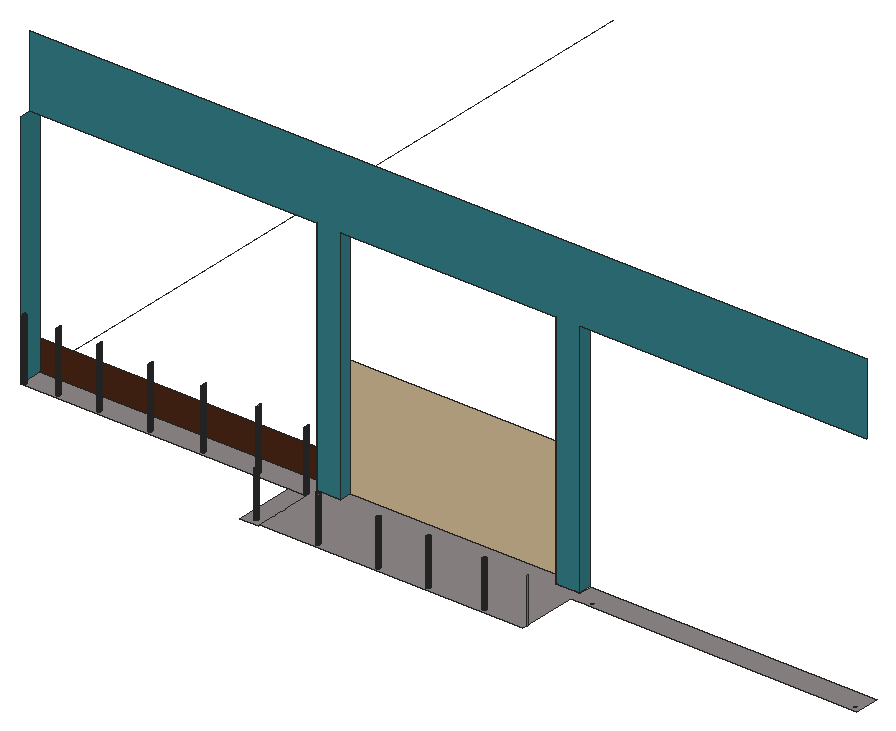
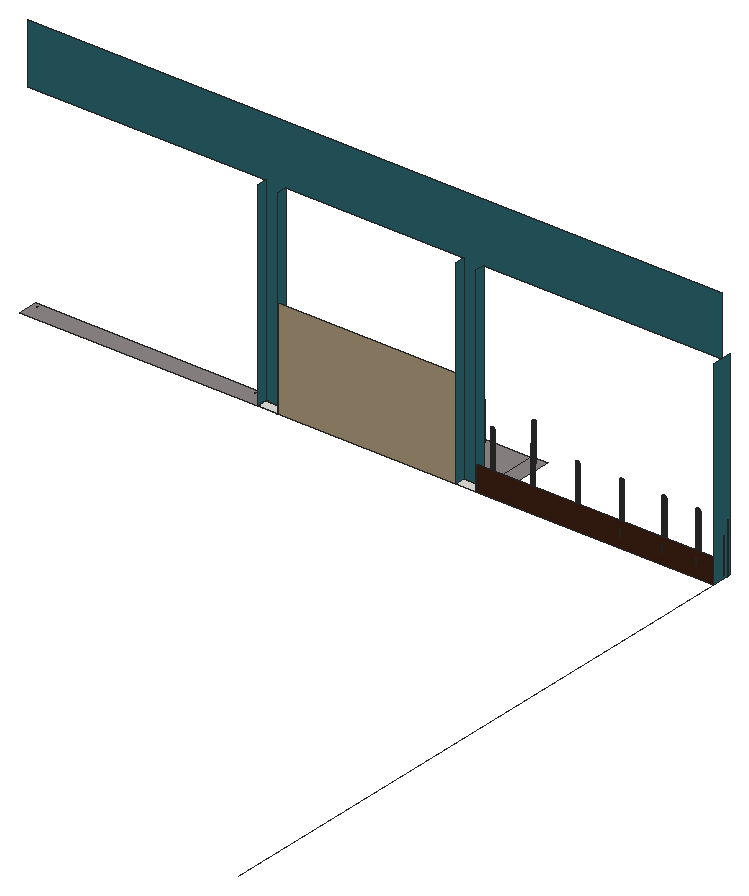
# SketchUp Ruby script. Lengths in inches.
U = 1.inch
M = Sketchup.active_model
def pt(a) = Geom::Point3d.new(a.map { |v| v * U })
def face(e, loops, mat)
  f = e.add_face(loops[0].map { |a| pt(a) })
  loops[1..].each { |l| e.add_face(l.map { |a| pt(a) }).erase! }
  f.material = f.back_material = mat if mat
  f
end
# faces: each face lists its corners as indices into pts; further lists are holes
def faces(e, pts, list, mat = nil) = list.each { |f| face(e, (f[0].is_a?(Array) ? f : [f]).map { |l| l.map { |i| pts[i] } }, mat) }
# xy, xz, yz: faces in a plane at the given z, y or x. An outline is a flat list of corners, or four numbers for a rectangle; further outlines are holes
def ring(l) = l.size == 4 ? [[l[0], l[1]], [l[2], l[1]], [l[2], l[3]], [l[0], l[3]]] : l.each_slice(2).to_a
def flat(e, list, mat, &to3) = list.each { |f| face(e, (f[0].is_a?(Array) ? f : [f]).map { |l| ring(l).map { |u, v| to3.(u, v) } }, mat) }
def xy(e, z, list, mat = nil) = flat(e, list, mat) { |x, y| [x, y, z] }
def xz(e, y, list, mat = nil) = flat(e, list, mat) { |x, z| [x, y, z] }
def yz(e, x, list, mat = nil) = flat(e, list, mat) { |y, z| [x, y, z] }
def lines(e, pts, list) = list.each { |a, b| e.add_line(pt(pts[a]), pt(pts[b])) }
# prism: a flat outline (further loops are holes) pulled along v
def prism(e, loops, v, mat = nil)
  f = face(e, loops, mat); d = Geom::Vector3d.new(v.map { |x| x * U })
  f.pushpull(f.normal.samedirection?(d) ? d.length : -d.length)
end
def box(e, o, s, mat = nil) = prism(e, [[o, [o[0] + s[0], o[1], o[2]], [o[0] + s[0], o[1] + s[1], o[2]], [o[0], o[1] + s[1], o[2]]]], [0, 0, s[2]], mat)
def at(x, y, z, deg = 0) = Geom::Transformation.translation(pt([x, y, z])) * Geom::Transformation.rotation(ORIGIN, Z_AXIS, deg.degrees)
def axes(o, x, y, z) = Geom::Transformation.new([*x, 0, *y, 0, *z, 0, *pt(o).to_a, 1])
def part(name) = M.definitions.add(name)
# library, detail: a bought-in or finely detailed component or shape, given as its bounding box
def library(name, o, s) = part(name).tap { |d| box(d.entities, o, s) }
def detail(e, o, s) = box(e.add_group.entities, o, s)
def put(e, d, t, mat = nil) = e.add_instance(d, t).tap { |i| i.material = mat if mat }
def group(e, t, mat = nil) = e.add_group.tap { |g| g.transformation = t; g.material = mat if mat }.entities
root = M.entities
M.materials.add("[0032_Moccasin]").color = [214, 191, 152]
M.materials.add("[0042_Sienna]").color = [76, 39, 21]
M.materials.add("[0083_DarkTurquoise]").color = [52, 127, 137]
M.materials.add("[Steel Brushed Stainless]").color = [183, 187, 190]
M.materials.add("[Stone Marble]").color = [143, 138, 136]
xy(root,167.95,[[648,109.2,672,121.2]])
xy(root,168,[[404.47,98.37,403.95,98.43,403.47,98.63,403.06,98.95,402.74,99.37,402.54,99.85,402.47,100.37,402.54,100.88,402.74,101.37,403.06,101.78,403.47,102.1,403.95,102.3,404.47,102.37,404.99,102.3,405.47,102.1,405.89,101.78,406.2,101.37,406.4,100.88,406.47,100.37,406.4,99.85,406.2,99.37,405.89,98.95,405.47,98.63,404.99,98.43],[408,109.2,432,121.2],[648,109.2,672,121.2]])
xy(root,168,[[[389.3,36.24,408,97.2],[400.07,41.47,399.55,41.54,399.07,41.74,398.65,42.05,398.33,42.47,398.13,42.95,398.07,43.47,398.13,43.99,398.33,44.47,398.65,44.88,399.07,45.2,399.55,45.4,400.07,45.47,400.58,45.4,401.07,45.2,401.48,44.88,401.8,44.47,402,43.99,402.07,43.47,402,42.95,401.8,42.47,401.48,42.05,401.07,41.74,400.58,41.54]],[[408,37.2,672,37.2,672,98.16,690.7,98.16,690.7,97.2,960,97.2,960,121.2,672,121.2,672,109.2,648,109.2,648,121.2,432,121.2,432,109.2,408,109.2,408,121.2,120,121.2,120,100.88,120.2,101.37,120.52,101.78,120.93,102.1,121.41,102.3,121.93,102.37,122.45,102.3,122.93,102.1,123.35,101.78,123.66,101.37,123.86,100.88,123.93,100.37,123.86,99.85,123.66,99.37,123.35,98.95,122.93,98.63,122.45,98.43,121.93,98.37,121.41,98.43,120.93,98.63,120.52,98.95,120.2,99.37,120,99.85,120,97.2,408,97.2],[954.01,100.13,953.77,100.17,953.53,100.2,953.51,100.21,953.49,100.21,953.05,100.39,953.03,100.41,953.01,100.41,952.82,100.5625,952.63,100.7,952.62,100.72,952.6,100.74,952.46,100.93,952.31,101.12,952.3,101.14,952.29,101.15,952.2,101.375,952.1,101.6,952.1,101.62,952.09,101.64,952.0625,101.875,952.03,102.11,952.03,102.16,952.0625,102.39,952.09,102.63,952.1,102.65,952.1,102.67,952.2,102.89,952.29,103.12,952.3,103.13,952.31,103.15,952.46,103.34,952.6,103.53,952.63,103.56,953.01,103.86,953.03,103.86,953.05,103.88,953.27,103.97,953.49,104.0625,953.51,104.0625,953.53,104.07,954.01,104.13,954.05,104.13,954.29,104.1,954.52,104.07,954.55,104.0625,954.57,104.0625,954.79,103.97,955.01,103.88,955.03,103.86,955.05,103.86,955.43,103.56,955.46,103.53,955.6,103.34,955.75,103.15,955.76,103.13,955.77,103.12,955.86,102.89,955.95,102.67,955.97,102.63,955.99,102.39,956.03,102.16,956.03,102.11,955.99,101.875,955.97,101.64,955.95,101.6,955.77,101.15,955.76,101.14,955.75,101.12,955.6,100.93,955.46,100.74,955.44,100.72,955.43,100.7,955.24,100.5625,955.05,100.41,955.03,100.41,955.01,100.39,954.57,100.21,954.55,100.21,954.52,100.2,954.29,100.17,954.05,100.13,954.03,100.14],[690.43,100.13,689.91,100.2,689.42,100.39,689.01,100.7,688.68,101.12,688.48,101.6,688.4,102.11,688.47,102.63,688.66,103.12,688.97,103.53,689.38,103.86,689.86,104.0625,690.38,104.13,690.9,104.07,691.38,103.88,691.8,103.56,692.125,103.15,692.33,102.67,692.4,102.16,692.34,101.64,692.15,101.15,691.83,100.74,691.42,100.41,690.94,100.21],[404.47,98.37,403.95,98.43,403.47,98.63,403.06,98.95,402.74,99.37,402.54,99.85,402.47,100.37,402.54,100.88,402.74,101.37,403.06,101.78,403.47,102.1,403.95,102.3,404.47,102.37,404.99,102.3,405.47,102.1,405.89,101.78,406.2,101.37,406.4,100.88,406.47,100.37,406.4,99.85,406.2,99.37,405.89,98.95,405.47,98.63,404.99,98.43]],[400.07,41.47,399.55,41.54,399.07,41.74,398.65,42.05,398.33,42.47,398.13,42.95,398.07,43.47,398.13,43.99,398.33,44.47,398.65,44.88,399.07,45.2,399.55,45.4,400.07,45.47,400.58,45.4,401.07,45.2,401.48,44.88,401.8,44.47,402,43.99,402.07,43.47,402,42.95,401.8,42.47,401.48,42.05,401.07,41.74,400.58,41.54]],"[Stone Marble]")
xz(root,109.2,[[648,167.95,672,168]])
xz(root,109.2,[[408,168,432,168,432,408,648,408,648,168,672,168,672,408,960,408,960,480,120,480,120,408,408,408]],"[0083_DarkTurquoise]")
xz(root,121.2,[[648,167.95,672,168]])
xz(root,121.2,[[432,168,648,288]],"[0032_Moccasin]")
xz(root,121.2,[[120,168,408,198]],"[0042_Sienna]")
yz(root,120,[[97.2,168,121.2,408]],"[0083_DarkTurquoise]")
yz(root,408,[[109.2,168,121.2,408]],"[0083_DarkTurquoise]")
yz(root,432,[[109.2,168,121.2,408]],"[0083_DarkTurquoise]")
yz(root,648,[[109.2,167.95,121.2,168]])
yz(root,648,[[109.2,168,121.2,408]],"[0083_DarkTurquoise]")
yz(root,672,[[109.2,167.95,121.2,168]])
yz(root,672,[[109.2,168,121.2,408]],"[0083_DarkTurquoise]")
p = [[461.31,41.04,168],[461.79,40.84,168],[461.79,40.84,213.56],[461.31,41.04,213.56],[462.31,40.78,168],[462.31,40.78,213.56],
  [462.83,40.84,168],[462.83,40.84,213.56],[463.31,41.04,168],[463.31,41.04,213.56],[522.25,41.04,168],[522.73,40.84,168],
  [522.73,40.84,213.56],[522.25,41.04,213.56],[523.25,40.78,168],[523.25,40.78,213.56],[523.76,40.84,168],[523.76,40.84,213.56],
  [524.25,41.04,168],[524.25,41.04,213.56],[572.31,41.04,168],[572.79,40.84,168],[572.79,40.84,213.56],[572.31,41.04,213.56],
  [573.31,40.78,168],[573.31,40.78,213.56],[573.83,40.84,168],[573.83,40.84,213.56],[574.31,41.04,168],[574.31,41.04,213.56],
  [628.68,41.04,168],[629.17,40.84,168],[629.17,40.84,213.56],[628.68,41.04,213.56],[629.68,40.78,168],[629.68,40.78,213.56],
  [630.2,40.84,168],[630.2,40.84,213.56],[630.68,41.04,168],[630.68,41.04,213.56],[460.89,41.36,168],[460.89,41.36,213.56],
  [463.72,41.36,168],[463.72,41.36,213.56],[521.83,41.36,168],[521.83,41.36,213.56],[524.66,41.36,168],[524.66,41.36,213.56],
  [571.89,41.36,168],[571.89,41.36,213.56],[574.72,41.36,168],[574.72,41.36,213.56],[628.27,41.36,168],[628.27,41.36,213.56],
  [631.1,41.36,168],[631.1,41.36,213.56],[460.58,41.78,168],[460.58,41.78,213.56],[464.04,41.78,168],[464.04,41.78,213.56],
  [521.51,41.78,168],[521.51,41.78,213.56],[524.98,41.78,168],[524.98,41.78,213.56],[571.58,41.78,168],[571.58,41.78,213.56],
  [575.04,41.78,168],[575.04,41.78,213.56],[627.95,41.78,168],[627.95,41.78,213.56],[631.41,41.78,168],[631.41,41.78,213.56],
  [399.07,41.74,168],[399.55,41.54,168],[399.55,41.54,213.19],[399.07,41.74,213.19],[400.07,41.47,168],[400.07,41.47,213.19],
  [400.58,41.54,168],[400.58,41.54,213.19],[401.07,41.74,168],[401.07,41.74,213.19],[398.65,42.05,168],[398.65,42.05,213.19],
  [401.48,42.05,168],[401.48,42.05,213.19],[460.375,42.26,168],[460.375,42.26,213.56],[464.24,42.26,168],[464.24,42.26,213.56],
  [521.3125,42.26,168],[521.3125,42.26,213.56],[525.18,42.26,168],[525.18,42.26,213.56],[571.375,42.26,168],[571.375,42.26,213.56],
  [575.24,42.26,168],[575.24,42.26,213.56],[627.75,42.26,168],[627.75,42.26,213.56],[631.61,42.26,168],[631.61,42.26,213.56],
  [398.33,42.47,168],[398.33,42.47,213.19],[401.8,42.47,168],[401.8,42.47,213.19],[460.31,42.78,168],[460.31,42.78,213.56],
  [464.31,42.78,168],[464.31,42.78,213.56],[521.25,42.78,168],[521.25,42.78,213.56],[525.25,42.78,168],[525.25,42.78,213.56],
  [571.31,42.78,168],[571.31,42.78,213.56],[575.31,42.78,168],[575.31,42.78,213.56],[627.68,42.78,168],[627.68,42.78,213.56],
  [631.68,42.78,168],[631.68,42.78,213.56],[672.75,42.78,168],[672.8125,42.26,168],[672.8125,42.26,213.56],[672.75,42.78,213.56],
  [398.13,42.95,168],[398.13,42.95,213.19],[402,42.95,168],[402,42.95,213.19],[460.375,43.29,168],[460.375,43.29,213.56],
  [464.24,43.29,168],[464.24,43.29,213.56],[521.3125,43.29,168],[521.3125,43.29,213.56],[525.18,43.29,168],[525.18,43.29,213.56],
  [571.375,43.29,168],[571.375,43.29,213.56],[575.24,43.29,168],[575.24,43.29,213.56],[627.75,43.29,168],[627.75,43.29,213.56],
  [631.61,43.29,168],[631.61,43.29,213.56],[672.8125,43.29,168],[672.8125,43.29,213.56],[398.07,43.47,168],[398.07,43.47,213.19],
  [402.07,43.47,168],[402.07,43.47,213.19],[460.58,43.78,168],[460.58,43.78,213.56],[464.04,43.78,168],[464.04,43.78,213.56],
  [521.51,43.78,168],[521.51,43.78,213.56],[524.98,43.78,168],[524.98,43.78,213.56],[571.58,43.78,168],[571.58,43.78,213.56],
  [575.04,43.78,168],[575.04,43.78,213.56],[627.95,43.78,168],[627.95,43.78,213.56],[631.41,43.78,168],[631.41,43.78,213.56],
  [398.13,43.99,168],[398.13,43.99,213.19],[402,43.99,168],[402,43.99,213.19],[460.89,44.19,168],[460.89,44.19,213.56],
  [463.72,44.19,168],[463.72,44.19,213.56],[521.83,44.19,168],[521.83,44.19,213.56],[524.66,44.19,168],[524.66,44.19,213.56],
  [571.89,44.19,168],[571.89,44.19,213.56],[574.72,44.19,168],[574.72,44.19,213.56],[628.27,44.19,168],[628.27,44.19,213.56],
  [631.1,44.19,168],[631.1,44.19,213.56],[398.33,44.47,168],[398.33,44.47,213.19],[401.8,44.47,168],[401.8,44.47,213.19],
  [461.31,44.51,168],[461.31,44.51,213.56],[463.31,44.51,168],[463.31,44.51,213.56],[522.25,44.51,168],[522.25,44.51,213.56],
  [524.25,44.51,168],[524.25,44.51,213.56],[572.31,44.51,168],[572.31,44.51,213.56],[574.31,44.51,168],[574.31,44.51,213.56],
  [628.68,44.51,168],[628.68,44.51,213.56],[630.68,44.51,168],[630.68,44.51,213.56],[398.65,44.88,168],[398.65,44.88,213.19],
  [401.48,44.88,168],[401.48,44.88,213.19],[461.79,44.71,168],[461.79,44.71,213.56],[462.83,44.71,168],[462.83,44.71,213.56],
  [522.73,44.71,168],[522.73,44.71,213.56],[523.76,44.71,168],[523.76,44.71,213.56],[572.79,44.71,168],[572.79,44.71,213.56],
  [573.83,44.71,168],[573.83,44.71,213.56],[629.17,44.71,168],[629.17,44.71,213.56],[630.2,44.71,168],[630.2,44.71,213.56],
  [462.31,44.78,168],[462.31,44.78,213.56],[523.25,44.78,168],[523.25,44.78,213.56],[573.31,44.78,168],[573.31,44.78,213.56],
  [629.68,44.78,168],[629.68,44.78,213.56],[399.07,45.2,168],[399.07,45.2,213.19],[401.07,45.2,168],[401.07,45.2,213.19],
  [399.55,45.4,168],[399.55,45.4,213.19],[400.58,45.4,168],[400.58,45.4,213.19],[400.07,45.47,168],[400.07,45.47,213.19],
  [121.41,98.43,228.52],[120.93,98.63,229],[120.93,98.63,168],[121.41,98.43,168],[121.93,98.37,228],[121.93,98.37,168],
  [122.45,98.43,227.48],[122.45,98.43,168],[122.93,98.63,227],[122.93,98.63,168],[403.47,98.63,168],[403.95,98.43,168],
  [403.95,98.43,227.48],[403.47,98.63,227],[404.47,98.37,168],[404.47,98.37,228],[404.99,98.43,168],[404.99,98.43,228.52],
  [405.47,98.63,168],[405.47,98.63,229],[120.52,98.95,229.41],[120.52,98.95,168],[123.35,98.95,226.59],[123.35,98.95,168],
  [403.06,98.95,168],[403.06,98.95,226.59],[405.89,98.95,168],[405.89,98.95,229.41],[120.2,99.37,229.73],[120.2,99.37,168],
  [123.66,99.37,226.27],[123.66,99.37,168],[402.74,99.37,168],[402.74,99.37,226.27],[406.2,99.37,168],[406.2,99.37,229.73],
  [120,99.85,229.93],[120,99.85,168],[123.86,99.85,226.07],[123.86,99.85,168],[402.54,99.85,168],[402.54,99.85,226.07],
  [406.4,99.85,168],[406.4,99.85,229.93],[119.93,100.37,230],[119.93,100.37,168],[123.93,100.37,226],[123.93,100.37,168],
  [402.47,100.37,168],[402.47,100.37,226],[406.47,100.37,168],[406.47,100.37,230],[154.07,100.13,227.98],[153.55,100.21,227.46],
  [153.55,100.21,168],[153.57,100.21,168],[153.83,100.17,168],[154.07,100.13,168],[154.59,100.2,228.5],[154.09,100.14,168],
  [154.35,100.17,168],[154.59,100.2,168],[195.19,100.13,227.98],[194.68,100.21,227.46],[194.68,100.21,168],[194.7,100.21,168],
  [194.96,100.17,168],[195.19,100.13,168],[195.71,100.2,228.5],[195.22,100.14,168],[195.47,100.17,168],[195.71,100.2,168],
  [246.26,100.13,227.98],[245.74,100.21,227.46],[245.74,100.21,168],[245.76,100.21,168],[246.02,100.17,168],[246.26,100.13,168],
  [246.77,100.2,228.5],[246.28,100.14,168],[246.54,100.17,168],[246.77,100.2,168],[299.94,100.13,227.98],[299.43,100.21,227.46],
  [299.43,100.21,168],[299.45,100.21,168],[299.71,100.17,168],[299.94,100.13,168],[300.46,100.2,228.5],[299.97,100.14,168],
  [300.22,100.17,168],[300.46,100.2,168],[354.57,100.13,227.98],[354.05,100.21,227.46],[354.05,100.21,168],[354.07,100.21,168],
  [354.33,100.17,168],[354.57,100.13,168],[355.09,100.2,228.5],[354.59,100.14,168],[354.85,100.17,168],[355.09,100.2,168],
  [153.07,100.41,226.98],[153.07,100.41,168],[153.09,100.41,168],[153.33,100.3,168],[155.07,100.39,228.98],[154.61,100.21,168],
  [154.85,100.3,168],[155.07,100.39,168],[194.2,100.41,226.98],[194.2,100.41,168],[194.22,100.41,168],[194.46,100.3,168],
  [196.2,100.39,228.98],[195.73,100.21,168],[195.97,100.3,168],[196.2,100.39,168],[245.26,100.41,226.98],[245.26,100.41,168],
  [245.28,100.41,168],[245.52,100.3,168],[247.26,100.39,228.98],[246.8,100.21,168],[247.04,100.3,168],[247.26,100.39,168],
  [298.95,100.41,226.98],[298.95,100.41,168],[298.97,100.41,168],[299.21,100.3,168],[300.95,100.39,228.98],[300.48,100.21,168],
  [300.72,100.3,168],[300.95,100.39,168],[353.57,100.41,226.98],[353.57,100.41,168],[353.59,100.41,168],[353.83,100.3,168],
  [355.57,100.39,228.98],[355.11,100.21,168],[355.35,100.3,168],[355.57,100.39,168],[120,100.88,229.93],[120,100.88,168],
  [123.86,100.88,226.07],[123.86,100.88,168],[152.66,100.74,226.57],[152.66,100.74,168],[152.68,100.72,168],[152.88,100.5625,168],
  [155.49,100.7,229.4],[155.09,100.41,168],[155.3,100.5625,168],[155.49,100.7,168],[193.79,100.74,226.57],[193.79,100.74,168],
  [193.8,100.72,168],[194.01,100.5625,168],[196.61,100.7,229.4],[196.21,100.41,168],[196.42,100.5625,168],[196.61,100.7,168],
  [244.85,100.74,226.57],[244.85,100.74,168],[244.87,100.72,168],[245.07,100.5625,168],[247.68,100.7,229.4],[247.28,100.41,168],
  [247.49,100.5625,168],[247.68,100.7,168],[298.54,100.74,226.57],[298.54,100.74,168],[298.55,100.72,168],[298.76,100.5625,168],
  [301.36,100.7,229.4],[300.96,100.41,168],[301.17,100.5625,168],[301.36,100.7,168],[353.16,100.74,226.57],[353.16,100.74,168],
  [353.18,100.72,168],[353.38,100.5625,168],[355.99,100.7,229.4],[355.59,100.41,168],[355.8,100.5625,168],[355.99,100.7,168],
  [402.54,100.88,168],[402.54,100.88,226.07],[406.4,100.88,168],[406.4,100.88,229.93],[152.35,101.15,226.26],[152.35,101.15,168],
  [152.36,101.14,168],[152.52,100.93,168],[155.8125,101.12,229.72],[155.5,100.72,168],[155.66,100.93,168],[155.8125,101.12,168],
  [193.47,101.15,226.26],[193.47,101.15,168],[193.49,101.14,168],[193.64,100.93,168],[196.9375,101.12,229.72],[196.63,100.72,168],
  [196.79,100.93,168],[196.9375,101.12,168],[244.54,101.15,226.26],[244.54,101.15,168],[244.55,101.14,168],[244.71,100.93,168],
  [248,101.12,229.72],[247.69,100.72,168],[247.85,100.93,168],[248,101.12,168],[298.22,101.15,226.26],[298.22,101.15,168],
  [298.24,101.14,168],[298.39,100.93,168],[301.6875,101.12,229.72],[301.38,100.72,168],[301.54,100.93,168],[301.6875,101.12,168],
  [352.85,101.15,226.26],[352.85,101.15,168],[352.86,101.14,168],[353.02,100.93,168],[356.3125,101.12,229.72],[356,100.72,168],
  [356.16,100.93,168],[356.3125,101.12,168],[120.2,101.37,229.73],[120.2,101.37,168],[123.66,101.37,226.27],[123.66,101.37,168],
  [402.74,101.37,168],[402.74,101.37,226.27],[406.2,101.37,168],[406.2,101.37,229.73],[156.02,101.6,229.93],[155.82,101.14,168],
  [155.92,101.375,168],[156.02,101.6,168],[197.14,101.6,229.93],[196.95,101.14,168],[197.05,101.375,168],[197.14,101.6,168],
  [248.2,101.6,229.93],[248.01,101.14,168],[248.11,101.375,168],[248.2,101.6,168],[301.89,101.6,229.93],[301.7,101.14,168],
  [301.8,101.375,168],[301.89,101.6,168],[356.52,101.6,229.93],[356.32,101.14,168],[356.42,101.375,168],[356.52,101.6,168],
  [152.15,101.64,226.0625],[152.15,101.64,168],[152.16,101.62,168],[152.26,101.375,168],[193.28,101.64,226.0625],[193.28,101.64,168],
  [193.29,101.62,168],[193.38,101.375,168],[244.34,101.64,226.0625],[244.34,101.64,168],[244.35,101.62,168],[244.45,101.375,168],
  [298.03,101.64,226.0625],[298.03,101.64,168],[298.04,101.62,168],[298.13,101.375,168],[352.65,101.64,226.0625],[352.65,101.64,168],
  [352.66,101.62,168],[352.76,101.375,168],[120.52,101.78,229.41],[120.52,101.78,168],[123.35,101.78,226.59],[123.35,101.78,168],
  [403.06,101.78,168],[403.06,101.78,226.59],[405.89,101.78,168],[405.89,101.78,229.41],[152.09,102.16,226],[152.09,102.16,168],
  [152.09,102.13,168],[152.125,101.875,168],[156.09,102.11,230],[156.02,101.62,168],[156.06,101.875,168],[156.09,102.11,168],
  [193.22,102.16,226],[193.22,102.16,168],[193.22,102.13,168],[193.25,101.875,168],[197.22,102.11,230],[197.15,101.62,168],
  [197.18,101.875,168],[197.22,102.11,168],[244.28,102.16,226],[244.28,102.16,168],[244.28,102.13,168],[244.3125,101.875,168],
  [248.28,102.11,230],[248.21,101.62,168],[248.24,101.875,168],[248.28,102.11,168],[297.97,102.16,226],[297.97,102.16,168],
  [297.97,102.13,168],[298,101.875,168],[301.97,102.11,230],[301.9,101.62,168],[301.93,101.875,168],[301.97,102.11,168],
  [352.59,102.16,226],[352.59,102.16,168],[352.59,102.13,168],[352.625,101.875,168],[356.59,102.11,230],[356.52,101.62,168],
  [356.56,101.875,168],[356.59,102.11,168],[120.93,102.1,229],[120.93,102.1,168],[122.93,102.1,227],[122.93,102.1,168],
  [403.47,102.1,168],[403.47,102.1,227],[405.47,102.1,168],[405.47,102.1,229],[121.41,102.3,228.52],[121.41,102.3,168],
  [122.45,102.3,227.48],[122.45,102.3,168],[156.03,102.63,229.9375],[156.09,102.13,168],[156.06,102.39,168],[156.03,102.63,168],
  [197.15,102.63,229.9375],[197.21,102.13,168],[197.18,102.39,168],[197.15,102.63,168],[248.22,102.63,229.9375],[248.28,102.13,168],
  [248.24,102.39,168],[248.22,102.63,168],[301.9,102.63,229.9375],[301.96,102.13,168],[301.93,102.39,168],[301.9,102.63,168],
  [356.53,102.63,229.9375],[356.59,102.13,168],[356.56,102.39,168],[356.53,102.63,168],[403.95,102.3,168],[403.95,102.3,227.48],
  [404.99,102.3,168],[404.99,102.3,228.52],[152.16,102.67,226.07],[152.16,102.67,168],[152.16,102.65,168],[152.125,102.39,168],
  [193.29,102.67,226.07],[193.29,102.67,168],[193.29,102.65,168],[193.25,102.39,168],[244.35,102.67,226.07],[244.35,102.67,168],
  [244.35,102.65,168],[244.3125,102.39,168],[298.04,102.67,226.07],[298.04,102.67,168],[298.04,102.65,168],[298,102.39,168],
  [352.66,102.67,226.07],[352.66,102.67,168],[352.66,102.65,168],[352.625,102.39,168],[121.93,102.37,228],[121.93,102.37,168],
  [404.47,102.37,168],[404.47,102.37,228],[155.83,103.12,229.74],[156.02,102.65,168],[155.92,102.89,168],[155.83,103.12,168],
  [196.96,103.12,229.74],[197.15,102.65,168],[197.05,102.89,168],[196.96,103.12,168],[248.02,103.12,229.74],[248.21,102.65,168],
  [248.11,102.89,168],[248.02,103.12,168],[301.71,103.12,229.74],[301.9,102.65,168],[301.8,102.89,168],[301.71,103.12,168],
  [356.33,103.12,229.74],[356.52,102.65,168],[356.42,102.89,168],[356.33,103.12,168],[152.37,103.15,226.28],[152.37,103.15,168],
  [152.36,103.13,168],[152.26,102.89,168],[193.5,103.15,226.28],[193.5,103.15,168],[193.49,103.13,168],[193.38,102.89,168],
  [244.56,103.15,226.28],[244.56,103.15,168],[244.55,103.13,168],[244.45,102.89,168],[298.25,103.15,226.28],[298.25,103.15,168],
  [298.24,103.13,168],[298.13,102.89,168],[352.87,103.15,226.28],[352.87,103.15,168],[352.86,103.13,168],[352.76,102.89,168],
  [155.52,103.53,229.43],[155.82,103.13,168],[155.66,103.34,168],[155.52,103.53,168],[196.65,103.53,229.43],[196.95,103.13,168],
  [196.79,103.34,168],[196.65,103.53,168],[247.71,103.53,229.43],[248.01,103.13,168],[247.85,103.34,168],[247.71,103.53,168],
  [301.4,103.53,229.43],[301.7,103.13,168],[301.54,103.34,168],[301.4,103.53,168],[356.02,103.53,229.43],[356.32,103.13,168],
  [356.16,103.34,168],[356.02,103.53,168],[152.69,103.56,226.6],[152.69,103.56,168],[152.68,103.55,168],[152.52,103.34,168],
  [193.82,103.56,226.6],[193.82,103.56,168],[193.8,103.55,168],[193.64,103.34,168],[244.88,103.56,226.6],[244.88,103.56,168],
  [244.87,103.55,168],[244.71,103.34,168],[298.57,103.56,226.6],[298.57,103.56,168],[298.55,103.55,168],[298.39,103.34,168],
  [353.19,103.56,226.6],[353.19,103.56,168],[353.18,103.55,168],[353.02,103.34,168],[155.11,103.86,229.02],[155.5,103.55,168],
  [155.3,103.71,168],[155.11,103.86,168],[196.24,103.86,229.02],[196.63,103.55,168],[196.42,103.71,168],[196.24,103.86,168],
  [247.3,103.86,229.02],[247.69,103.55,168],[247.49,103.71,168],[247.3,103.86,168],[300.99,103.86,229.02],[301.38,103.55,168],
  [301.17,103.71,168],[300.99,103.86,168],[355.61,103.86,229.02],[356,103.55,168],[355.8,103.71,168],[355.61,103.86,168],
  [153.11,103.88,227.02],[153.11,103.88,168],[153.09,103.86,168],[152.88,103.71,168],[194.24,103.88,227.02],[194.24,103.88,168],
  [194.22,103.86,168],[194.01,103.71,168],[245.3,103.88,227.02],[245.3,103.88,168],[245.28,103.86,168],[245.07,103.71,168],
  [298.99,103.88,227.02],[298.99,103.88,168],[298.97,103.86,168],[298.76,103.71,168],[353.61,103.88,227.02],[353.61,103.88,168],
  [353.59,103.86,168],[353.38,103.71,168],[153.59,104.07,227.5],[153.59,104.07,168],[153.57,104.0625,168],[153.33,103.97,168],
  [154.63,104.0625,228.54],[155.09,103.86,168],[154.85,103.97,168],[154.63,104.0625,168],[194.72,104.07,227.5],[194.72,104.07,168],
  [194.7,104.0625,168],[194.46,103.97,168],[195.76,104.0625,228.54],[196.21,103.86,168],[195.97,103.97,168],[195.76,104.0625,168],
  [245.78,104.07,227.5],[245.78,104.07,168],[245.76,104.0625,168],[245.52,103.97,168],[246.82,104.0625,228.54],[247.28,103.86,168],
  [247.04,103.97,168],[246.82,104.0625,168],[299.47,104.07,227.5],[299.47,104.07,168],[299.45,104.0625,168],[299.21,103.97,168],
  [300.51,104.0625,228.54],[300.96,103.86,168],[300.72,103.97,168],[300.51,104.0625,168],[354.09,104.07,227.5],[354.09,104.07,168],
  [354.07,104.0625,168],[353.83,103.97,168],[355.13,104.0625,228.54],[355.59,103.86,168],[355.35,103.97,168],[355.13,104.0625,168],
  [154.11,104.13,228.02],[154.11,104.13,168],[154.09,104.13,168],[153.83,104.1,168],[154.61,104.0625,168],[154.35,104.1,168],
  [195.24,104.13,228.02],[195.24,104.13,168],[195.22,104.13,168],[194.96,104.1,168],[195.73,104.0625,168],[195.47,104.1,168],
  [246.3,104.13,228.02],[246.3,104.13,168],[246.28,104.13,168],[246.02,104.1,168],[246.8,104.0625,168],[246.54,104.1,168],
  [299.99,104.13,228.02],[299.99,104.13,168],[299.97,104.13,168],[299.71,104.1,168],[300.48,104.0625,168],[300.22,104.1,168],
  [354.61,104.13,228.02],[354.61,104.13,168],[354.59,104.13,168],[354.33,104.1,168],[355.11,104.0625,168],[354.85,104.1,168],
  [120,841.2,168],[120,121.2,168],[404.47,100.37,168],[404.47,100.37,228],[121.93,100.37,168],[121.93,100.37,228],
  [400.07,43.47,213.19],[400.07,43.47,168]]
faces(root,p,[[0,1,2,3],[1,4,5,2],[4,6,7,5],[6,8,9,7],[10,11,12,13],[11,14,15,12],[14,16,17,15],[16,18,19,17],
  [20,21,22,23],[21,24,25,22],[24,26,27,25],[26,28,29,27],[30,31,32,33],[31,34,35,32],[34,36,37,35],[36,38,39,37],
  [40,0,3,41],[8,42,43,9],[44,10,13,45],[18,46,47,19],[48,20,23,49],[28,50,51,29],[52,30,33,53],[38,54,55,39],
  [56,40,41,57],[42,58,59,43],[60,44,45,61],[46,62,63,47],[64,48,49,65],[50,66,67,51],[68,52,53,69],[54,70,71,55],
  [72,73,74,75],[73,76,77,74],[76,78,79,77],[78,80,81,79],[82,72,75,83],[80,84,85,81],[86,56,57,87],[58,88,89,59],
  [90,60,61,91],[62,92,93,63],[94,64,65,95],[66,96,97,67],[98,68,69,99],[70,100,101,71],[102,82,83,103],[84,104,105,85],
  [106,86,87,107],[88,108,109,89],[110,90,91,111],[92,112,113,93],[114,94,95,115],[96,116,117,97],[118,98,99,119],[100,120,121,101],
  [122,123,124,125],[126,102,103,127],[104,128,129,105],[130,106,107,131],[108,132,133,109],[134,110,111,135],[112,136,137,113],[138,114,115,139],
  [116,140,141,117],[142,118,119,143],[120,144,145,121],[146,122,125,147],[148,126,127,149],[128,150,151,129],[152,130,131,153],[132,154,155,133],
  [156,134,135,157],[136,158,159,137],[160,138,139,161],[140,162,163,141],[164,142,143,165],[144,166,167,145],[168,148,149,169],[150,170,171,151],
  [172,152,153,173],[154,174,175,155],[176,156,157,177],[158,178,179,159],[180,160,161,181],[162,182,183,163],[184,164,165,185],[166,186,187,167],
  [188,168,169,189],[170,190,191,171],[192,172,173,193],[174,194,195,175],[196,176,177,197],[178,198,199,179],[200,180,181,201],[182,202,203,183],
  [204,184,185,205],[186,206,207,187],[208,188,189,209],[190,210,211,191],[212,192,193,213],[194,214,215,195],[216,196,197,217],[198,218,219,199],
  [220,200,201,221],[202,222,223,203],[224,204,205,225],[206,226,227,207],[228,212,213,229],[214,228,229,215],[230,216,217,231],[218,230,231,219],
  [232,220,221,233],[222,232,233,223],[234,224,225,235],[226,234,235,227],[236,208,209,237],[210,238,239,211],[240,236,237,241],[238,242,243,239],
  [244,240,241,245],[242,244,245,243]],"[Stone Marble]")
faces(root,p,[[246,247,248,249],[250,246,249,251],[252,250,251,253],[254,252,253,255],[256,257,258,259],[257,260,261,258],[260,262,263,261],[262,264,265,263],
  [247,266,267,248],[268,254,255,269],[270,256,259,271],[264,272,273,265],[266,274,275,267],[276,268,269,277],[278,270,271,279],[272,280,281,273],
  [274,282,283,275],[284,276,277,285],[286,278,279,287],[280,288,289,281],[282,290,291,283],[292,284,285,293],[294,286,287,295],[288,296,297,289],
  [298,299,300,301,302,303],[304,298,303,305,306,307],[308,309,310,311,312,313],[314,308,313,315,316,317],[318,319,320,321,322,323],[324,318,323,325,326,327],[328,329,330,331,332,333],[334,328,333,335,336,337],
  [338,339,340,341,342,343],[344,338,343,345,346,347],[299,348,349,350,351,300],[352,304,307,353,354,355],[309,356,357,358,359,310],[360,314,317,361,362,363],[319,364,365,366,367,320],[368,324,327,369,370,371],
  [329,372,373,374,375,330],[376,334,337,377,378,379],[339,380,381,382,383,340],[384,344,347,385,386,387],[290,388,389,291],[390,292,293,391],[348,392,393,394,395,349],[396,352,355,397,398,399],
  [356,400,401,402,403,357],[404,360,363,405,406,407],[364,408,409,410,411,365],[412,368,371,413,414,415],[372,416,417,418,419,373],[420,376,379,421,422,423],[380,424,425,426,427,381],[428,384,387,429,430,431],
  [432,294,295,433],[296,434,435,297],[392,436,437,438,439,393],[440,396,399,441,442,443],[400,444,445,446,447,401],[448,404,407,449,450,451],[408,452,453,454,455,409],[456,412,415,457,458,459],
  [416,460,461,462,463,417],[464,420,423,465,466,467],[424,468,469,470,471,425],[472,428,431,473,474,475],[388,476,477,389],[478,390,391,479],[480,432,433,481],[434,482,483,435],
  [484,440,443,485,486,487],[488,448,451,489,490,491],[492,456,459,493,494,495],[496,464,467,497,498,499],[500,472,475,501,502,503],[436,504,505,506,507,437],[444,508,509,510,511,445],[452,512,513,514,515,453],
  [460,516,517,518,519,461],[468,520,521,522,523,469],[476,524,525,477],[526,478,479,527],[528,480,481,529],[482,530,531,483],[504,532,533,534,535,505],[536,484,487,537,538,539],
  [508,540,541,542,543,509],[544,488,491,545,546,547],[512,548,549,550,551,513],[552,492,495,553,554,555],[516,556,557,558,559,517],[560,496,499,561,562,563],[520,564,565,566,567,521],[568,500,503,569,570,571],
  [524,572,573,525],[574,526,527,575],[576,528,529,577],[530,578,579,531],[572,580,581,573],[582,574,575,583],[584,536,539,585,586,587],[588,544,547,589,590,591],
  [592,552,555,593,594,595],[596,560,563,597,598,599],[600,568,571,601,602,603],[604,576,577,605],[578,606,607,579],[532,608,609,610,611,533],[540,612,613,614,615,541],[548,616,617,618,619,549],
  [556,620,621,622,623,557],[564,624,625,626,627,565],[580,628,629,581],[628,582,583,629],[630,604,605,631],[606,630,631,607],[632,584,587,633,634,635],[636,588,591,637,638,639],
  [640,592,595,641,642,643],[644,596,599,645,646,647],[648,600,603,649,650,651],[608,652,653,654,655,609],[612,656,657,658,659,613],[616,660,661,662,663,617],[620,664,665,666,667,621],[624,668,669,670,671,625],
  [672,632,635,673,674,675],[676,636,639,677,678,679],[680,640,643,681,682,683],[684,644,647,685,686,687],[688,648,651,689,690,691],[652,692,693,694,695,653],[656,696,697,698,699,657],[660,700,701,702,703,661],
  [664,704,705,706,707,665],[668,708,709,710,711,669],[712,672,675,713,714,715],[716,676,679,717,718,719],[720,680,683,721,722,723],[724,684,687,725,726,727],[728,688,691,729,730,731],[692,732,733,734,735,693],
  [696,736,737,738,739,697],[700,740,741,742,743,701],[704,744,745,746,747,705],[708,748,749,750,751,709],[732,752,753,754,755,733],[756,712,715,757,758,759],[736,760,761,762,763,737],[764,716,719,765,766,767],
  [740,768,769,770,771,741],[772,720,723,773,774,775],[744,776,777,778,779,745],[780,724,727,781,782,783],[748,784,785,786,787,749],[788,728,731,789,790,791],[752,792,793,794,795,753],[792,756,759,796,797,793],
  [760,798,799,800,801,761],[798,764,767,802,803,799],[768,804,805,806,807,769],[804,772,775,808,809,805],[776,810,811,812,813,777],[810,780,783,814,815,811],[784,816,817,818,819,785],[816,788,791,820,821,817]],"[Steel Brushed Stainless]")
lines(root,p,[[822,823],[824,825],[826,827],[828,829]])
